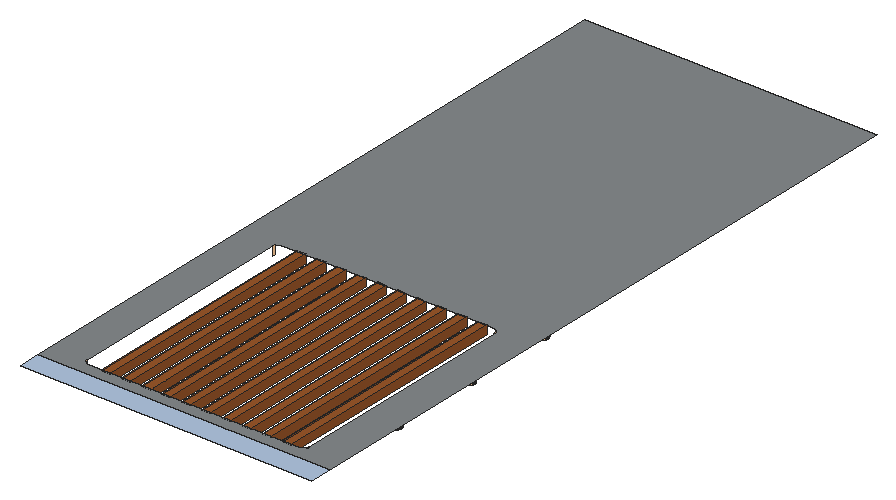
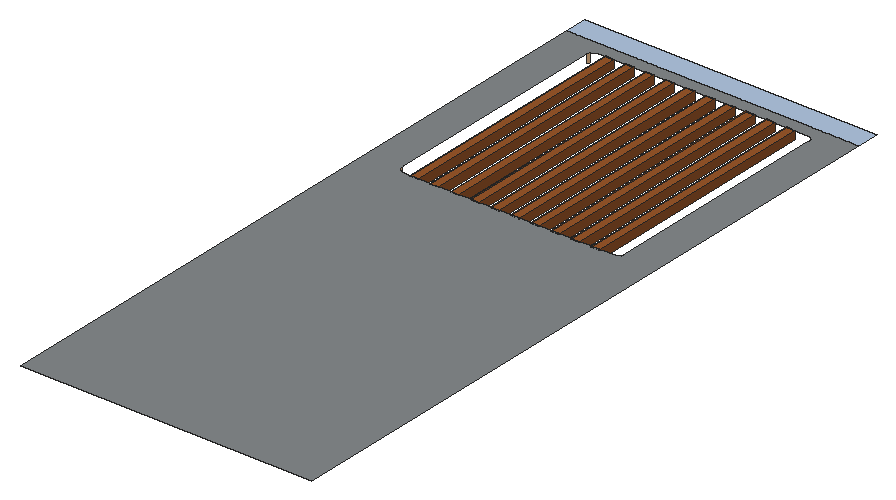
# SketchUp Ruby script. Lengths in inches.
U = 1.inch
M = Sketchup.active_model
def pt(a) = Geom::Point3d.new(a.map { |v| v * U })
def face(e, loops, mat)
  f = e.add_face(loops[0].map { |a| pt(a) })
  loops[1..].each { |l| e.add_face(l.map { |a| pt(a) }).erase! }
  f.material = f.back_material = mat if mat
  f
end
# faces: each face lists its corners as indices into pts; further lists are holes
def faces(e, pts, list, mat = nil) = list.each { |f| face(e, (f[0].is_a?(Array) ? f : [f]).map { |l| l.map { |i| pts[i] } }, mat) }
# xy, xz, yz: faces in a plane at the given z, y or x. An outline is a flat list of corners, or four numbers for a rectangle; further outlines are holes
def ring(l) = l.size == 4 ? [[l[0], l[1]], [l[2], l[1]], [l[2], l[3]], [l[0], l[3]]] : l.each_slice(2).to_a
def flat(e, list, mat, &to3) = list.each { |f| face(e, (f[0].is_a?(Array) ? f : [f]).map { |l| ring(l).map { |u, v| to3.(u, v) } }, mat) }
def xy(e, z, list, mat = nil) = flat(e, list, mat) { |x, y| [x, y, z] }
def xz(e, y, list, mat = nil) = flat(e, list, mat) { |x, z| [x, y, z] }
def yz(e, x, list, mat = nil) = flat(e, list, mat) { |y, z| [x, y, z] }
def lines(e, pts, list) = list.each { |a, b| e.add_line(pt(pts[a]), pt(pts[b])) }
# prism: a flat outline (further loops are holes) pulled along v
def prism(e, loops, v, mat = nil)
  f = face(e, loops, mat); d = Geom::Vector3d.new(v.map { |x| x * U })
  f.pushpull(f.normal.samedirection?(d) ? d.length : -d.length)
end
def box(e, o, s, mat = nil) = prism(e, [[o, [o[0] + s[0], o[1], o[2]], [o[0] + s[0], o[1] + s[1], o[2]], [o[0], o[1] + s[1], o[2]]]], [0, 0, s[2]], mat)
def at(x, y, z, deg = 0) = Geom::Transformation.translation(pt([x, y, z])) * Geom::Transformation.rotation(ORIGIN, Z_AXIS, deg.degrees)
def axes(o, x, y, z) = Geom::Transformation.new([*x, 0, *y, 0, *z, 0, *pt(o).to_a, 1])
def part(name) = M.definitions.add(name)
# library, detail: a bought-in or finely detailed component or shape, given as its bounding box
def library(name, o, s) = part(name).tap { |d| box(d.entities, o, s) }
def detail(e, o, s) = box(e.add_group.entities, o, s)
def put(e, d, t, mat = nil) = e.add_instance(d, t).tap { |i| i.material = mat if mat }
def group(e, t, mat = nil) = e.add_group.tap { |g| g.transformation = t; g.material = mat if mat }.entities
root = M.entities
M.materials.add("[0099_LightSteelBlue]").color = [176, 196, 222]
M.materials.add("[Blacktop Old 01]").color = [132, 136, 139]
M.materials.add("[Color C02]").color = [255, 204, 153]
M.materials.add("[Wood Cherry Original]").color = [152, 86, 42]
c1 = part("Group\#14")
box(c1.entities,[0,-170.54,0],[6,170.54,6])
xy(root,373,[[193.29,138.77,192.52,138.9,191.8125,139.23,191.21,139.74,190.76,140.38,190.5,141.12,190.43,141.9,190.57,142.67,190.9,143.38,191.4,143.98,192.04,144.43,192.78,144.69,193.56,144.76,194.33,144.625,195.04,144.29,195.64,143.79,196.09,143.15,196.36,142.41,196.42,141.63,196.29,140.86,195.95,140.15,195.45,139.55,194.81,139.1,194.07,138.83],[11.87,139.23,11.1,139.37,10.39,139.7,9.79,140.21,9.34,140.85,9.07,141.58,9,142.36,9.14,143.14,9.47,143.85,9.98,144.44,10.62,144.89,11.35,145.16,12.13,145.23,12.9,145.09,13.61,144.76,14.21,144.26,14.66,143.61,14.93,142.88,15,142.1,14.86,141.33,14.53,140.62,14.02,140.02,13.38,139.57,12.65,139.3],[196.29,195.4,195.52,195.54,194.8125,195.87,194.21,196.375,193.76,197.02,193.5,197.75,193.43,198.53,193.57,199.3,193.9,200.01,194.4,200.61,195.04,201.0625,195.78,201.33,196.56,201.4,197.33,201.26,198.04,200.93,198.64,200.42,199.09,199.78,199.36,199.05,199.42,198.27,199.29,197.49,198.95,196.78,198.45,196.19,197.81,195.74,197.07,195.47],[11.87,198.88,11.1,199.02,10.39,199.35,9.79,199.85,9.34,200.49,9.07,201.23,9,202.01,9.14,202.78,9.47,203.49,9.98,204.09,10.62,204.54,11.35,204.81,12.13,204.875,12.9,204.74,13.61,204.41,14.21,203.9,14.66,203.26,14.93,202.52,15,201.74,14.86,200.97,14.53,200.26,14.02,199.66,13.38,199.21,12.65,198.95],[11.87,258.53,11.1,258.66,10.39,258.99,9.79,259.5,9.34,260.14,9.07,260.875,9,261.66,9.14,262.43,9.47,263.14,9.98,263.74,10.62,264.19,11.35,264.45,12.13,264.52,12.9,264.38,13.61,264.05,14.21,263.55,14.66,262.91,14.93,262.17,15,261.39,14.86,260.62,14.53,259.91,14.02,259.31,13.38,258.86,12.65,258.59],
  [196.29,259.4,195.52,259.54,194.8125,259.87,194.21,260.375,193.76,261.02,193.5,261.75,193.43,262.53,193.57,263.3,193.9,264.01,194.4,264.61,195.04,265.0625,195.78,265.33,196.56,265.4,197.33,265.26,198.04,264.93,198.64,264.42,199.09,263.78,199.36,263.05,199.42,262.27,199.29,261.49,198.95,260.78,198.45,260.19,197.81,259.74,197.07,259.47],[11.87,318.17,11.1,318.31,10.39,318.64,9.79,319.14,9.34,319.79,9.07,320.52,9,321.3,9.14,322.07,9.47,322.78,9.98,323.38,10.62,323.83,11.35,324.1,12.13,324.17,12.9,324.03,13.61,323.7,14.21,323.19,14.66,322.55,14.93,321.82,15,321.04,14.86,320.26,14.53,319.55,14.02,318.96,13.38,318.51,12.65,318.24],[73.34,319.91,72.57,320.05,71.86,320.38,71.26,320.89,70.8125,321.53,70.55,322.27,70.48,323.05,70.61,323.82,70.95,324.53,71.45,325.125,72.09,325.57,72.83,325.84,73.61,325.91,74.38,325.77,75.09,325.44,75.6875,324.9375,76.14,324.29,76.4,323.56,76.47,322.78,76.34,322.01,76,321.3,75.5,320.7,74.86,320.25,74.12,319.98],[134.82,321.66,134.05,321.79,133.34,322.125,132.74,322.63,132.29,323.27,132.02,324.01,131.95,324.79,132.09,325.56,132.42,326.27,132.93,326.87,133.57,327.32,134.3,327.58,135.08,327.65,135.86,327.52,136.56,327.18,137.16,326.68,137.61,326.04,137.88,325.3,137.95,324.52,137.8125,323.75,137.48,323.04,136.98,322.44,136.33,321.99,135.6,321.73],[196.29,323.4,195.52,323.54,194.8125,323.87,194.21,324.375,193.76,325.02,193.5,325.75,193.43,326.53,193.57,327.3,193.9,328.01,194.4,328.61,195.04,329.0625,195.78,329.33,196.56,329.4,197.33,329.26,198.04,328.93,198.64,328.42,199.09,327.78,199.36,327.05,199.42,326.27,199.29,325.49,198.95,324.78,198.45,324.19,197.81,323.74,197.07,323.47]],"[Color C02]")
xy(root,378,[[0,114.625,203.78,130.0625]],"[0099_LightSteelBlue]")
xy(root,378,[[[0,130.0625,203.78,607.58],[30,138.625,28.17,138.79,26.67,139.29,25.5,140.125,24.67,141.29,24.17,142.79,24,144.625,24,303.17,24.17,305,24.67,306.5,25.5,307.67,26.67,308.5,28.17,309,30,309.17,173.78,309.17,175.61,309,177.11,308.5,178.28,307.67,179.11,306.5,179.61,305,179.78,303.17,179.78,144.625,179.61,142.79,179.11,141.29,178.28,140.125,177.11,139.29,175.61,138.79,173.78,138.625]]],"[Blacktop Old 01]")
p = [[193.29,138.77,372],[192.52,138.9,372],[192.52,138.9,373],[193.29,138.77,373],[194.07,138.83,372],[194.07,138.83,373],
  [194.81,139.1,372],[194.81,139.1,373],[191.8125,139.23,372],[191.8125,139.23,373],[195.45,139.55,372],[195.45,139.55,373],
  [11.87,139.23,372],[11.1,139.37,372],[11.1,139.37,373],[11.87,139.23,373],[12.65,139.3,372],[12.65,139.3,373],
  [191.21,139.74,372],[191.21,139.74,373],[13.38,139.57,372],[13.38,139.57,373],[10.39,139.7,372],[10.39,139.7,373],
  [195.95,140.15,372],[195.95,140.15,373],[14.02,140.02,372],[14.02,140.02,373],[9.79,140.21,372],[9.79,140.21,373],
  [190.76,140.38,372],[190.76,140.38,373],[14.53,140.62,372],[14.53,140.62,373],[196.29,140.86,372],[196.29,140.86,373],
  [9.34,140.85,372],[9.34,140.85,373],[190.5,141.12,372],[190.5,141.12,373],[14.86,141.33,372],[14.86,141.33,373],
  [9.07,141.58,372],[9.07,141.58,373],[196.42,141.63,372],[196.42,141.63,373],[190.43,141.9,372],[190.43,141.9,373],
  [15,142.1,372],[15,142.1,373],[24.17,142.79,372],[24.17,142.79,378],[24.67,141.29,378],[24.67,141.29,372],
  [179.61,142.79,378],[179.61,142.79,372],[179.11,141.29,372],[179.11,141.29,378],[9,142.36,372],[9,142.36,373],
  [196.36,142.41,372],[196.36,142.41,373],[190.57,142.67,372],[190.57,142.67,373],[14.93,142.88,372],[14.93,142.88,373],
  [9.14,143.14,372],[9.14,143.14,373],[196.09,143.15,372],[196.09,143.15,373],[190.9,143.38,372],[190.9,143.38,373],
  [14.66,143.61,372],[14.66,143.61,373],[9.47,143.85,372],[9.47,143.85,373],[195.64,143.79,372],[195.64,143.79,373],
  [191.4,143.98,372],[191.4,143.98,373],[14.21,144.26,372],[14.21,144.26,373],[9.98,144.44,372],[9.98,144.44,373],
  [195.04,144.29,372],[195.04,144.29,373],[192.04,144.43,372],[192.04,144.43,373],[13.61,144.76,372],[13.61,144.76,373],
  [194.33,144.625,372],[194.33,144.625,373],[10.62,144.89,372],[10.62,144.89,373],[192.78,144.69,372],[192.78,144.69,373],
  [193.56,144.76,372],[193.56,144.76,373],[12.9,145.09,372],[12.9,145.09,373],[11.35,145.16,372],[11.35,145.16,373],
  [12.13,145.23,372],[12.13,145.23,373],[196.29,195.4,372],[195.52,195.54,372],[195.52,195.54,373],[196.29,195.4,373],
  [197.07,195.47,372],[197.07,195.47,373],[194.8125,195.87,372],[194.8125,195.87,373],[197.81,195.74,372],[197.81,195.74,373],
  [198.45,196.19,372],[198.45,196.19,373],[194.21,196.375,372],[194.21,196.375,373],[198.95,196.78,372],[198.95,196.78,373],
  [193.76,197.02,372],[193.76,197.02,373],[199.29,197.49,372],[199.29,197.49,373],[193.5,197.75,372],[193.5,197.75,373],
  [199.42,198.27,372],[199.42,198.27,373],[193.43,198.53,372],[193.43,198.53,373],[199.36,199.05,372],[199.36,199.05,373],
  [193.57,199.3,372],[193.57,199.3,373],[11.87,198.88,372],[11.1,199.02,372],[11.1,199.02,373],[11.87,198.88,373],
  [12.65,198.95,372],[12.65,198.95,373],[10.39,199.35,372],[10.39,199.35,373],[199.09,199.78,372],[199.09,199.78,373],
  [9.79,199.85,372],[9.79,199.85,373],[193.9,200.01,372],[193.9,200.01,373],[198.64,200.42,372],[198.64,200.42,373],
  [9.34,200.49,372],[9.34,200.49,373],[194.4,200.61,372],[194.4,200.61,373],[198.04,200.93,372],[198.04,200.93,373],
  [9.07,201.23,372],[9.07,201.23,373],[195.04,201.0625,372],[195.04,201.0625,373],[197.33,201.26,372],[197.33,201.26,373],
  [195.78,201.33,372],[195.78,201.33,373],[9,202.01,372],[9,202.01,373],[196.56,201.4,372],[196.56,201.4,373],
  [9.14,202.78,372],[9.14,202.78,373],[9.47,203.49,372],[9.47,203.49,373],[9.98,204.09,372],[9.98,204.09,373],
  [10.62,204.54,372],[10.62,204.54,373],[12.9,204.74,372],[13.61,204.41,372],[13.61,204.41,373],[12.9,204.74,373],
  [11.35,204.81,372],[11.35,204.81,373],[12.13,204.875,372],[12.13,204.875,373],[196.29,259.4,372],[195.52,259.54,372],
  [195.52,259.54,373],[196.29,259.4,373],[197.07,259.47,372],[197.07,259.47,373],[194.8125,259.87,372],[194.8125,259.87,373],
  [197.81,259.74,372],[197.81,259.74,373],[198.45,260.19,372],[198.45,260.19,373],[194.21,260.375,372],[194.21,260.375,373],
  [198.95,260.78,372],[198.95,260.78,373],[193.76,261.02,372],[193.76,261.02,373],[199.29,261.49,372],[199.29,261.49,373],
  [193.5,261.75,372],[193.5,261.75,373],[199.42,262.27,372],[199.42,262.27,373],[193.43,262.53,372],[193.43,262.53,373],
  [199.36,263.05,372],[199.36,263.05,373],[193.57,263.3,372],[193.57,263.3,373],[199.09,263.78,372],[199.09,263.78,373],
  [193.9,264.01,372],[193.9,264.01,373],[198.64,264.42,372],[198.64,264.42,373],[194.4,264.61,372],[194.4,264.61,373],
  [198.04,264.93,372],[198.04,264.93,373],[195.04,265.0625,372],[195.04,265.0625,373],[197.33,265.26,372],[197.33,265.26,373],
  [195.78,265.33,372],[195.78,265.33,373],[196.56,265.4,372],[196.56,265.4,373],[24.17,305,378],[24.17,305,372],
  [24.67,306.5,372],[24.67,306.5,378],[179.61,305,372],[179.61,305,378],[179.11,306.5,378],[179.11,306.5,372],
  [134.82,321.66,372],[134.05,321.79,372],[134.05,321.79,373],[134.82,321.66,373],[135.6,321.73,372],[135.6,321.73,373],
  [136.33,321.99,372],[136.33,321.99,373],[133.34,322.125,372],[133.34,322.125,373],[136.98,322.44,372],[136.98,322.44,373],
  [132.74,322.63,372],[132.74,322.63,373],[137.48,323.04,372],[137.48,323.04,373],[132.29,323.27,372],[132.29,323.27,373],
  [137.8125,323.75,372],[137.8125,323.75,373],[132.02,324.01,372],[132.02,324.01,373],[196.29,323.4,372],[195.52,323.54,372],
  [195.52,323.54,373],[196.29,323.4,373],[197.07,323.47,372],[197.07,323.47,373],[194.8125,323.87,372],[194.8125,323.87,373],
  [197.81,323.74,372],[197.81,323.74,373],[198.45,324.19,372],[198.45,324.19,373],[137.95,324.52,372],[137.95,324.52,373],
  [194.21,324.375,372],[194.21,324.375,373],[131.95,324.79,372],[131.95,324.79,373],[198.95,324.78,372],[198.95,324.78,373],
  [193.76,325.02,372],[193.76,325.02,373],[137.88,325.3,372],[137.88,325.3,373],[132.09,325.56,372],[132.09,325.56,373],
  [199.29,325.49,372],[199.29,325.49,373],[193.5,325.75,372],[193.5,325.75,373],[137.61,326.04,372],[137.61,326.04,373],
  [199.42,326.27,372],[199.42,326.27,373],[132.42,326.27,372],[132.42,326.27,373],[193.43,326.53,372],[193.43,326.53,373],
  [137.16,326.68,372],[137.16,326.68,373],[132.93,326.87,372],[132.93,326.87,373],[199.36,327.05,372],[199.36,327.05,373],
  [193.57,327.3,372],[193.57,327.3,373],[136.56,327.18,372],[136.56,327.18,373],[133.57,327.32,372],[133.57,327.32,373],
  [199.09,327.78,372],[199.09,327.78,373],[135.86,327.52,372],[135.86,327.52,373],[134.3,327.58,372],[134.3,327.58,373],
  [193.9,328.01,372],[193.9,328.01,373],[135.08,327.65,372],[135.08,327.65,373],[198.64,328.42,372],[198.64,328.42,373],
  [194.4,328.61,372],[194.4,328.61,373],[198.04,328.93,372],[198.04,328.93,373],[195.04,329.0625,372],[195.04,329.0625,373],
  [197.33,329.26,372],[197.33,329.26,373],[195.78,329.33,372],[195.78,329.33,373],[196.56,329.4,372],[196.56,329.4,373]]
faces(root,p,[[0,1,2,3],[4,0,3,5],[6,4,5,7],[1,8,9,2],[10,6,7,11],[12,13,14,15],[16,12,15,17],[8,18,19,9],
  [20,16,17,21],[13,22,23,14],[24,10,11,25],[26,20,21,27],[22,28,29,23],[18,30,31,19],[32,26,27,33],[34,24,25,35],
  [28,36,37,29],[30,38,39,31],[40,32,33,41],[36,42,43,37],[44,34,35,45],[38,46,47,39],[48,40,41,49],[50,51,52,53],
  [54,55,56,57],[42,58,59,43],[60,44,45,61],[46,62,63,47],[64,48,49,65],[58,66,67,59],[68,60,61,69],[62,70,71,63],
  [72,64,65,73],[66,74,75,67],[76,68,69,77],[70,78,79,71],[80,72,73,81],[74,82,83,75],[84,76,77,85],[78,86,87,79],
  [88,80,81,89],[90,84,85,91],[82,92,93,83],[86,94,95,87],[96,90,91,97],[94,96,97,95],[98,88,89,99],[92,100,101,93],
  [102,98,99,103],[100,102,103,101],[104,105,106,107],[108,104,107,109],[105,110,111,106],[112,108,109,113],[114,112,113,115],[110,116,117,111],
  [118,114,115,119],[116,120,121,117],[122,118,119,123],[120,124,125,121],[126,122,123,127],[124,128,129,125],[130,126,127,131],[128,132,133,129],
  [134,135,136,137],[138,134,137,139],[135,140,141,136],[142,130,131,143],[140,144,145,141],[132,146,147,133],[148,142,143,149],[144,150,151,145],
  [146,152,153,147],[154,148,149,155],[150,156,157,151],[152,158,159,153],[160,154,155,161],[158,162,163,159],[156,164,165,157],[162,166,167,163],
  [166,160,161,167],[164,168,169,165],[168,170,171,169],[170,172,173,171],[172,174,175,173],[176,177,178,179],[174,180,181,175],[182,176,179,183],
  [180,182,183,181],[184,185,186,187],[188,184,187,189],[185,190,191,186],[192,188,189,193],[194,192,193,195],[190,196,197,191],[198,194,195,199],
  [196,200,201,197],[202,198,199,203],[200,204,205,201],[206,202,203,207],[204,208,209,205],[210,206,207,211],[208,212,213,209],[214,210,211,215],
  [212,216,217,213],[218,214,215,219],[216,220,221,217],[222,218,219,223],[220,224,225,221],[226,222,223,227],[224,228,229,225],[228,230,231,229],
  [230,226,227,231],[232,233,234,235],[236,237,238,239],[240,241,242,243],[244,240,243,245],[246,244,245,247],[241,248,249,242],[250,246,247,251],
  [248,252,253,249],[254,250,251,255],[252,256,257,253],[258,254,255,259],[256,260,261,257],[262,263,264,265],[266,262,265,267],[263,268,269,264],
  [270,266,267,271],[272,270,271,273],[274,258,259,275],[268,276,277,269],[260,278,279,261],[280,272,273,281],[276,282,283,277],[284,274,275,285],
  [278,286,287,279],[288,280,281,289],[282,290,291,283],[292,284,285,293],[294,288,289,295],[286,296,297,287],[290,298,299,291],[300,292,293,301],
  [296,302,303,297],[304,294,295,305],[298,306,307,299],[308,300,301,309],[302,310,311,303],[312,304,305,313],[314,308,309,315],[310,316,317,311],
  [306,318,319,307],[320,314,315,321],[316,320,321,317],[322,312,313,323],[318,324,325,319],[326,322,323,327],[324,328,329,325],[330,326,327,331],
  [328,332,333,329],[332,334,335,333],[334,330,331,335]],"[Color C02]")
put(root,c1,at(37.58,309.17,372),"[Wood Cherry Original]")
put(root,c1,at(51.65,309.17,372),"[Wood Cherry Original]")
put(root,c1,at(65.71,309.17,372),"[Wood Cherry Original]")
put(root,c1,at(79.77,309.17,372),"[Wood Cherry Original]")
put(root,c1,at(93.83,309.17,372),"[Wood Cherry Original]")
put(root,c1,at(107.9,309.17,372),"[Wood Cherry Original]")
put(root,c1,at(121.96,309.17,372),"[Wood Cherry Original]")
put(root,c1,at(136.02,309.17,372),"[Wood Cherry Original]")
put(root,c1,at(150.08,309.17,372),"[Wood Cherry Original]")
put(root,c1,at(164.15,309.17,372),"[Wood Cherry Original]")
